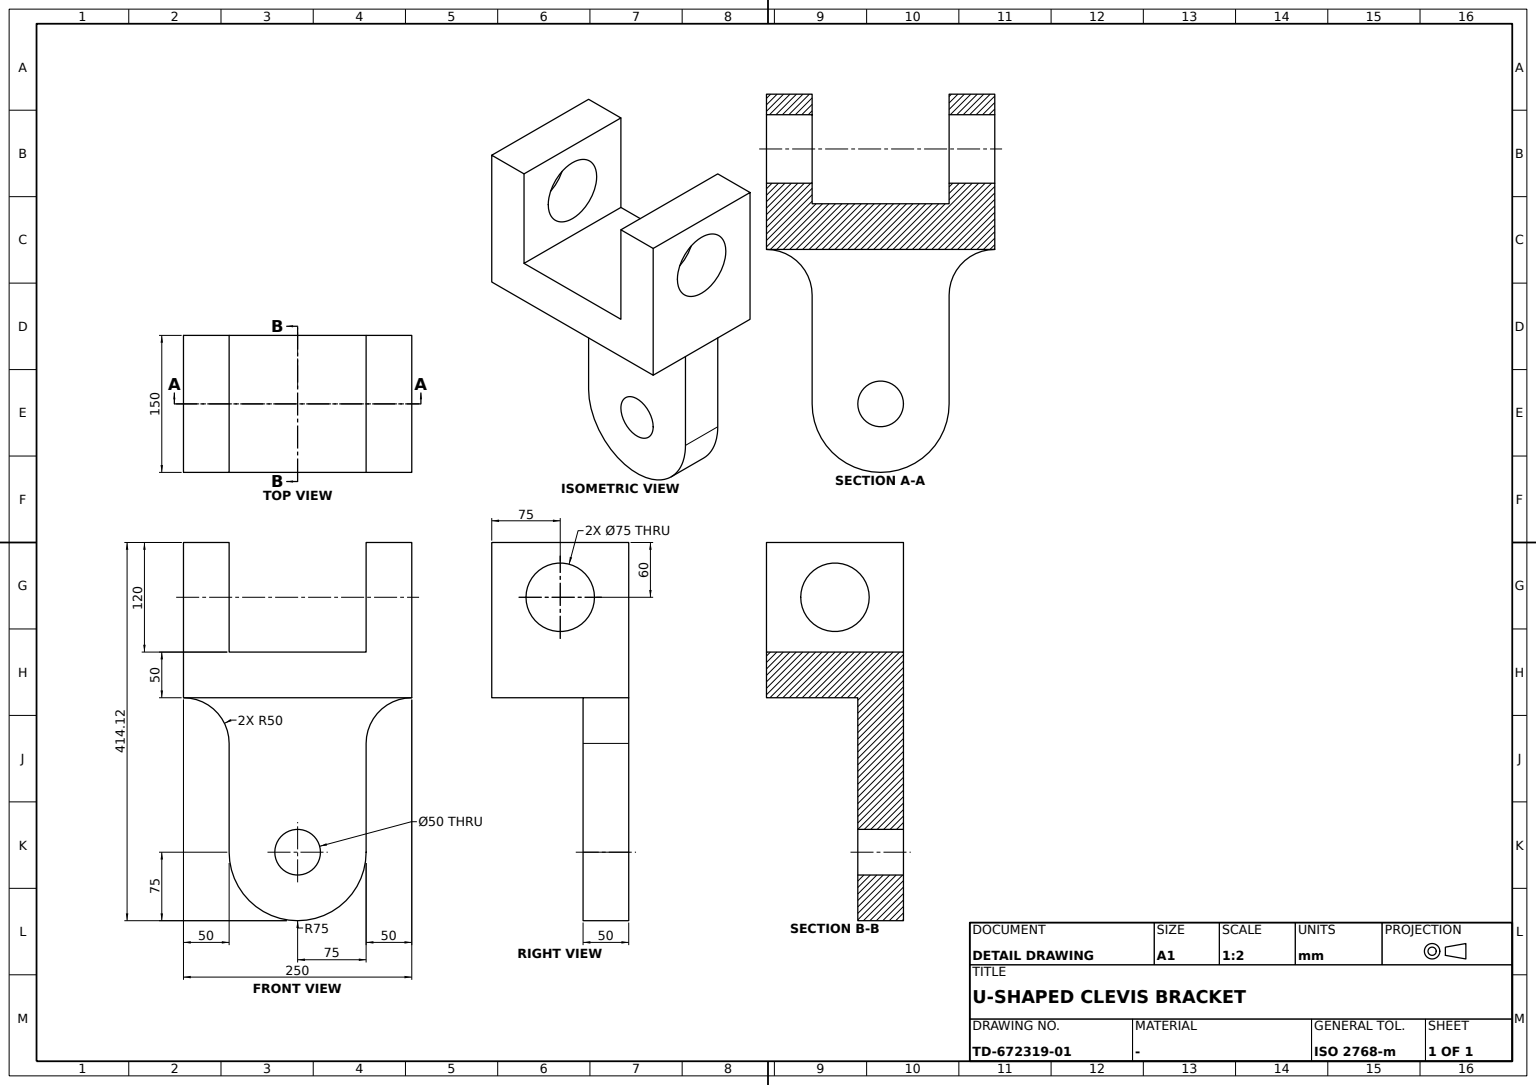
ISO-10303-21;
HEADER;
FILE_DESCRIPTION((''),'2;1');
FILE_NAME('','',(''),(''),'','','');
FILE_SCHEMA(('AUTOMOTIVE_DESIGN'));
ENDSEC;
DATA;
#1=APPLICATION_CONTEXT('');
#2=PRODUCT_CONTEXT('',#1,'mechanical');
#3=PRODUCT('','','',(#2));
#4=PRODUCT_DEFINITION_FORMATION('','',#3);
#5=PRODUCT_DEFINITION_CONTEXT('',#1,'design');
#6=PRODUCT_DEFINITION('','',#4,#5);
#7=PRODUCT_DEFINITION_SHAPE('','',#6);
#8=(LENGTH_UNIT()NAMED_UNIT(*)SI_UNIT(.MILLI.,.METRE.));
#9=(NAMED_UNIT(*)PLANE_ANGLE_UNIT()SI_UNIT($,.RADIAN.));
#10=(NAMED_UNIT(*)SI_UNIT($,.STERADIAN.)SOLID_ANGLE_UNIT());
#11=UNCERTAINTY_MEASURE_WITH_UNIT(LENGTH_MEASURE(1.E-05),#8,'distance_accuracy_value','');
#12=(GEOMETRIC_REPRESENTATION_CONTEXT(3)GLOBAL_UNCERTAINTY_ASSIGNED_CONTEXT((#11))GLOBAL_UNIT_ASSIGNED_CONTEXT((#8,#9,#10))REPRESENTATION_CONTEXT('',''));
#13=CARTESIAN_POINT('',(37.5,75.,60.));
#14=VERTEX_POINT('',#13);
#15=CARTESIAN_POINT('',(-37.5,75.,60.));
#16=VERTEX_POINT('',#15);
#17=CARTESIAN_POINT('',(0.,75.,60.));
#18=DIRECTION('',(0.,1.,0.));
#19=DIRECTION('',(0.,0.,1.));
#20=AXIS2_PLACEMENT_3D('',#17,#18,#19);
#21=CIRCLE('',#20,37.5);
#22=EDGE_CURVE('',#14,#16,#21,.T.);
#23=ORIENTED_EDGE('',*,*,#22,.F.);
#24=CARTESIAN_POINT('',(37.5,125.,60.));
#25=VERTEX_POINT('',#24);
#26=CARTESIAN_POINT('',(37.5,-0.66,60.));
#27=DIRECTION('',(0.,-1.,0.));
#28=VECTOR('',#27,1000.);
#29=LINE('',#26,#28);
#30=EDGE_CURVE('',#25,#14,#29,.T.);
#31=ORIENTED_EDGE('',*,*,#30,.F.);
#32=CARTESIAN_POINT('',(-37.5,125.,60.));
#33=VERTEX_POINT('',#32);
#34=CARTESIAN_POINT('',(0.,125.,60.));
#35=DIRECTION('',(-1.,0.,0.));
#36=AXIS2_PLACEMENT_3D('',#34,#18,#35);
#37=CIRCLE('',#36,37.5);
#38=EDGE_CURVE('',#25,#33,#37,.T.);
#39=ORIENTED_EDGE('',*,*,#38,.T.);
#40=CARTESIAN_POINT('',(-37.5,-0.66,60.));
#41=LINE('',#40,#28);
#42=EDGE_CURVE('',#33,#16,#41,.T.);
#43=ORIENTED_EDGE('',*,*,#42,.T.);
#44=EDGE_LOOP('',(#23,#31,#39,#43));
#45=FACE_OUTER_BOUND('',#44,.T.);
#46=CARTESIAN_POINT('',(0.,-0.66,60.));
#47=AXIS2_PLACEMENT_3D('',#46,#27,#35);
#48=CYLINDRICAL_SURFACE('',#47,37.5);
#49=ADVANCED_FACE('',(#45),#48,.F.);
#50=CARTESIAN_POINT('',(75.,-75.,0.));
#51=VERTEX_POINT('',#50);
#52=CARTESIAN_POINT('',(75.,-75.,120.));
#53=VERTEX_POINT('',#52);
#54=CARTESIAN_POINT('',(75.,-75.,60.));
#55=VECTOR('',#19,1000.);
#56=LINE('',#54,#55);
#57=EDGE_CURVE('',#51,#53,#56,.T.);
#58=ORIENTED_EDGE('',*,*,#57,.F.);
#59=CARTESIAN_POINT('',(-75.,-75.,0.));
#60=VERTEX_POINT('',#59);
#61=CARTESIAN_POINT('',(0.,-75.,0.));
#62=DIRECTION('',(1.,0.,0.));
#63=VECTOR('',#62,1000.);
#64=LINE('',#61,#63);
#65=EDGE_CURVE('',#60,#51,#64,.T.);
#66=ORIENTED_EDGE('',*,*,#65,.F.);
#67=CARTESIAN_POINT('',(-75.,-75.,120.));
#68=VERTEX_POINT('',#67);
#69=CARTESIAN_POINT('',(-75.,-75.,60.));
#70=LINE('',#69,#55);
#71=EDGE_CURVE('',#60,#68,#70,.T.);
#72=ORIENTED_EDGE('',*,*,#71,.T.);
#73=CARTESIAN_POINT('',(0.,-75.,120.));
#74=LINE('',#73,#63);
#75=EDGE_CURVE('',#68,#53,#74,.T.);
#76=ORIENTED_EDGE('',*,*,#75,.T.);
#77=EDGE_LOOP('',(#58,#66,#72,#76));
#78=FACE_OUTER_BOUND('',#77,.T.);
#79=CARTESIAN_POINT('',(-37.5,-75.,60.));
#80=VERTEX_POINT('',#79);
#81=CARTESIAN_POINT('',(37.5,-75.,60.));
#82=VERTEX_POINT('',#81);
#83=CARTESIAN_POINT('',(0.,-75.,60.));
#84=AXIS2_PLACEMENT_3D('',#83,#18,#19);
#85=CIRCLE('',#84,37.5);
#86=EDGE_CURVE('',#80,#82,#85,.T.);
#87=ORIENTED_EDGE('',*,*,#86,.F.);
#88=EDGE_CURVE('',#82,#80,#85,.T.);
#89=ORIENTED_EDGE('',*,*,#88,.F.);
#90=EDGE_LOOP('',(#87,#89));
#91=FACE_BOUND('',#90,.T.);
#92=AXIS2_PLACEMENT_3D('',#61,#18,#19);
#93=PLANE('',#92);
#94=ADVANCED_FACE('',(#78,#91),#93,.T.);
#95=ORIENTED_EDGE('',*,*,#38,.F.);
#96=EDGE_CURVE('',#33,#25,#37,.T.);
#97=ORIENTED_EDGE('',*,*,#96,.F.);
#98=EDGE_LOOP('',(#95,#97));
#99=FACE_BOUND('',#98,.T.);
#100=CARTESIAN_POINT('',(75.,125.,-50.));
#101=VERTEX_POINT('',#100);
#102=CARTESIAN_POINT('',(75.,125.,120.));
#103=VERTEX_POINT('',#102);
#104=CARTESIAN_POINT('',(75.,125.,35.));
#105=LINE('',#104,#55);
#106=EDGE_CURVE('',#101,#103,#105,.T.);
#107=ORIENTED_EDGE('',*,*,#106,.F.);
#108=CARTESIAN_POINT('',(-25.,125.,-50.));
#109=VERTEX_POINT('',#108);
#110=CARTESIAN_POINT('',(25.,125.,-50.));
#111=LINE('',#110,#63);
#112=EDGE_CURVE('',#109,#101,#111,.T.);
#113=ORIENTED_EDGE('',*,*,#112,.F.);
#114=CARTESIAN_POINT('',(-75.,125.,-50.));
#115=VERTEX_POINT('',#114);
#116=CARTESIAN_POINT('',(0.,125.,-50.));
#117=LINE('',#116,#63);
#118=EDGE_CURVE('',#115,#109,#117,.T.);
#119=ORIENTED_EDGE('',*,*,#118,.F.);
#120=CARTESIAN_POINT('',(-75.,125.,120.));
#121=VERTEX_POINT('',#120);
#122=CARTESIAN_POINT('',(-75.,125.,35.));
#123=LINE('',#122,#55);
#124=EDGE_CURVE('',#115,#121,#123,.T.);
#125=ORIENTED_EDGE('',*,*,#124,.T.);
#126=CARTESIAN_POINT('',(0.,125.,120.));
#127=LINE('',#126,#63);
#128=EDGE_CURVE('',#121,#103,#127,.T.);
#129=ORIENTED_EDGE('',*,*,#128,.T.);
#130=EDGE_LOOP('',(#107,#113,#119,#125,#129));
#131=FACE_OUTER_BOUND('',#130,.T.);
#132=DIRECTION('',(0.,0.,-1.));
#133=AXIS2_PLACEMENT_3D('',#126,#27,#132);
#134=PLANE('',#133);
#135=ADVANCED_FACE('',(#99,#131),#134,.F.);
#136=CARTESIAN_POINT('',(75.,75.,0.));
#137=VERTEX_POINT('',#136);
#138=CARTESIAN_POINT('',(75.,0.,0.));
#139=LINE('',#138,#28);
#140=EDGE_CURVE('',#137,#51,#139,.T.);
#141=ORIENTED_EDGE('',*,*,#140,.F.);
#142=CARTESIAN_POINT('',(-75.,75.,0.));
#143=VERTEX_POINT('',#142);
#144=CARTESIAN_POINT('',(0.,75.,0.));
#145=LINE('',#144,#63);
#146=EDGE_CURVE('',#143,#137,#145,.T.);
#147=ORIENTED_EDGE('',*,*,#146,.F.);
#148=CARTESIAN_POINT('',(-75.,0.,0.));
#149=LINE('',#148,#28);
#150=EDGE_CURVE('',#143,#60,#149,.T.);
#151=ORIENTED_EDGE('',*,*,#150,.T.);
#152=ORIENTED_EDGE('',*,*,#65,.T.);
#153=EDGE_LOOP('',(#141,#147,#151,#152));
#154=FACE_OUTER_BOUND('',#153,.T.);
#155=AXIS2_PLACEMENT_3D('',#61,#132,#18);
#156=PLANE('',#155);
#157=ADVANCED_FACE('',(#154),#156,.F.);
#158=CARTESIAN_POINT('',(-25.,-25.,-219.120758));
#159=VERTEX_POINT('',#158);
#160=CARTESIAN_POINT('',(-25.,25.,-219.120758));
#161=VERTEX_POINT('',#160);
#162=CARTESIAN_POINT('',(-25.,0.,-219.120758));
#163=AXIS2_PLACEMENT_3D('',#162,#62,#132);
#164=CIRCLE('',#163,25.);
#165=EDGE_CURVE('',#159,#161,#164,.T.);
#166=ORIENTED_EDGE('',*,*,#165,.T.);
#167=CARTESIAN_POINT('',(-75.,25.,-219.120758));
#168=VERTEX_POINT('',#167);
#169=CARTESIAN_POINT('',(0.,25.,-219.120758));
#170=LINE('',#169,#63);
#171=EDGE_CURVE('',#168,#161,#170,.T.);
#172=ORIENTED_EDGE('',*,*,#171,.F.);
#173=CARTESIAN_POINT('',(-75.,-25.,-219.120758));
#174=VERTEX_POINT('',#173);
#175=CARTESIAN_POINT('',(-75.,0.,-219.120758));
#176=AXIS2_PLACEMENT_3D('',#175,#62,#18);
#177=CIRCLE('',#176,25.);
#178=EDGE_CURVE('',#174,#168,#177,.T.);
#179=ORIENTED_EDGE('',*,*,#178,.F.);
#180=CARTESIAN_POINT('',(0.,-25.,-219.120758));
#181=LINE('',#180,#63);
#182=EDGE_CURVE('',#174,#159,#181,.T.);
#183=ORIENTED_EDGE('',*,*,#182,.T.);
#184=EDGE_LOOP('',(#166,#172,#179,#183));
#185=FACE_OUTER_BOUND('',#184,.T.);
#186=CARTESIAN_POINT('',(0.,0.,-219.120758));
#187=AXIS2_PLACEMENT_3D('',#186,#35,#18);
#188=CYLINDRICAL_SURFACE('',#187,25.);
#189=ADVANCED_FACE('',(#185),#188,.F.);
#190=CARTESIAN_POINT('',(-75.,75.,-219.120758));
#191=VERTEX_POINT('',#190);
#192=CARTESIAN_POINT('',(-25.,75.,-219.120758));
#193=VERTEX_POINT('',#192);
#194=CARTESIAN_POINT('',(0.,75.,-219.120758));
#195=LINE('',#194,#63);
#196=EDGE_CURVE('',#191,#193,#195,.T.);
#197=ORIENTED_EDGE('',*,*,#196,.F.);
#198=CARTESIAN_POINT('',(-75.,75.,-100.));
#199=VERTEX_POINT('',#198);
#200=CARTESIAN_POINT('',(-75.,75.,-159.560379));
#201=LINE('',#200,#55);
#202=EDGE_CURVE('',#191,#199,#201,.T.);
#203=ORIENTED_EDGE('',*,*,#202,.T.);
#204=CARTESIAN_POINT('',(-25.,75.,-100.));
#205=VERTEX_POINT('',#204);
#206=CARTESIAN_POINT('',(-50.,75.,-100.));
#207=LINE('',#206,#63);
#208=EDGE_CURVE('',#199,#205,#207,.T.);
#209=ORIENTED_EDGE('',*,*,#208,.T.);
#210=CARTESIAN_POINT('',(-25.,75.,-159.560379));
#211=LINE('',#210,#55);
#212=EDGE_CURVE('',#193,#205,#211,.T.);
#213=ORIENTED_EDGE('',*,*,#212,.F.);
#214=EDGE_LOOP('',(#197,#203,#209,#213));
#215=FACE_OUTER_BOUND('',#214,.T.);
#216=AXIS2_PLACEMENT_3D('',#194,#18,#19);
#217=PLANE('',#216);
#218=ADVANCED_FACE('',(#215),#217,.T.);
#219=CARTESIAN_POINT('',(-75.,-75.,-219.120758));
#220=VERTEX_POINT('',#219);
#221=CIRCLE('',#176,75.);
#222=EDGE_CURVE('',#220,#191,#221,.T.);
#223=ORIENTED_EDGE('',*,*,#222,.T.);
#224=ORIENTED_EDGE('',*,*,#196,.T.);
#225=CARTESIAN_POINT('',(-25.,-75.,-219.120758));
#226=VERTEX_POINT('',#225);
#227=CIRCLE('',#163,75.);
#228=EDGE_CURVE('',#226,#193,#227,.T.);
#229=ORIENTED_EDGE('',*,*,#228,.F.);
#230=CARTESIAN_POINT('',(-50.,-75.,-219.120758));
#231=LINE('',#230,#63);
#232=EDGE_CURVE('',#220,#226,#231,.T.);
#233=ORIENTED_EDGE('',*,*,#232,.F.);
#234=EDGE_LOOP('',(#223,#224,#229,#233));
#235=FACE_OUTER_BOUND('',#234,.T.);
#236=CYLINDRICAL_SURFACE('',#187,75.);
#237=ADVANCED_FACE('',(#235),#236,.T.);
#238=ORIENTED_EDGE('',*,*,#42,.F.);
#239=ORIENTED_EDGE('',*,*,#96,.T.);
#240=ORIENTED_EDGE('',*,*,#30,.T.);
#241=EDGE_CURVE('',#16,#14,#21,.T.);
#242=ORIENTED_EDGE('',*,*,#241,.F.);
#243=EDGE_LOOP('',(#238,#239,#240,#242));
#244=FACE_OUTER_BOUND('',#243,.T.);
#245=ADVANCED_FACE('',(#244),#48,.F.);
#246=ORIENTED_EDGE('',*,*,#140,.T.);
#247=ORIENTED_EDGE('',*,*,#57,.T.);
#248=CARTESIAN_POINT('',(75.,-125.,120.));
#249=VERTEX_POINT('',#248);
#250=CARTESIAN_POINT('',(75.,-100.,120.));
#251=LINE('',#250,#28);
#252=EDGE_CURVE('',#53,#249,#251,.T.);
#253=ORIENTED_EDGE('',*,*,#252,.T.);
#254=CARTESIAN_POINT('',(75.,-125.,-50.));
#255=VERTEX_POINT('',#254);
#256=CARTESIAN_POINT('',(75.,-125.,35.));
#257=VECTOR('',#132,1000.);
#258=LINE('',#256,#257);
#259=EDGE_CURVE('',#249,#255,#258,.T.);
#260=ORIENTED_EDGE('',*,*,#259,.T.);
#261=CARTESIAN_POINT('',(75.,0.,-50.));
#262=VECTOR('',#18,1000.);
#263=LINE('',#261,#262);
#264=EDGE_CURVE('',#255,#101,#263,.T.);
#265=ORIENTED_EDGE('',*,*,#264,.T.);
#266=ORIENTED_EDGE('',*,*,#106,.T.);
#267=CARTESIAN_POINT('',(75.,75.,120.));
#268=VERTEX_POINT('',#267);
#269=CARTESIAN_POINT('',(75.,100.,120.));
#270=LINE('',#269,#28);
#271=EDGE_CURVE('',#103,#268,#270,.T.);
#272=ORIENTED_EDGE('',*,*,#271,.T.);
#273=CARTESIAN_POINT('',(75.,75.,60.));
#274=LINE('',#273,#257);
#275=EDGE_CURVE('',#268,#137,#274,.T.);
#276=ORIENTED_EDGE('',*,*,#275,.T.);
#277=EDGE_LOOP('',(#246,#247,#253,#260,#265,#266,#272,#276));
#278=FACE_OUTER_BOUND('',#277,.T.);
#279=AXIS2_PLACEMENT_3D('',#138,#62,#18);
#280=PLANE('',#279);
#281=ADVANCED_FACE('',(#278),#280,.T.);
#282=ORIENTED_EDGE('',*,*,#271,.F.);
#283=ORIENTED_EDGE('',*,*,#128,.F.);
#284=CARTESIAN_POINT('',(-75.,75.,120.));
#285=VERTEX_POINT('',#284);
#286=CARTESIAN_POINT('',(-75.,100.,120.));
#287=LINE('',#286,#28);
#288=EDGE_CURVE('',#121,#285,#287,.T.);
#289=ORIENTED_EDGE('',*,*,#288,.T.);
#290=CARTESIAN_POINT('',(0.,75.,120.));
#291=LINE('',#290,#63);
#292=EDGE_CURVE('',#285,#268,#291,.T.);
#293=ORIENTED_EDGE('',*,*,#292,.T.);
#294=EDGE_LOOP('',(#282,#283,#289,#293));
#295=FACE_OUTER_BOUND('',#294,.T.);
#296=AXIS2_PLACEMENT_3D('',#73,#19,#27);
#297=PLANE('',#296);
#298=ADVANCED_FACE('',(#295),#297,.T.);
#299=CARTESIAN_POINT('',(-75.,-125.,120.));
#300=VERTEX_POINT('',#299);
#301=CARTESIAN_POINT('',(-75.,-100.,120.));
#302=LINE('',#301,#28);
#303=EDGE_CURVE('',#68,#300,#302,.T.);
#304=ORIENTED_EDGE('',*,*,#303,.F.);
#305=ORIENTED_EDGE('',*,*,#71,.F.);
#306=ORIENTED_EDGE('',*,*,#150,.F.);
#307=CARTESIAN_POINT('',(-75.,75.,60.));
#308=LINE('',#307,#257);
#309=EDGE_CURVE('',#285,#143,#308,.T.);
#310=ORIENTED_EDGE('',*,*,#309,.F.);
#311=ORIENTED_EDGE('',*,*,#288,.F.);
#312=ORIENTED_EDGE('',*,*,#124,.F.);
#313=CARTESIAN_POINT('',(-75.,125.,-100.));
#314=AXIS2_PLACEMENT_3D('',#313,#35,#18);
#315=CIRCLE('',#314,50.);
#316=EDGE_CURVE('',#199,#115,#315,.T.);
#317=ORIENTED_EDGE('',*,*,#316,.F.);
#318=ORIENTED_EDGE('',*,*,#202,.F.);
#319=ORIENTED_EDGE('',*,*,#222,.F.);
#320=CARTESIAN_POINT('',(-75.,-75.,-100.));
#321=VERTEX_POINT('',#320);
#322=CARTESIAN_POINT('',(-75.,-75.,-159.560379));
#323=LINE('',#322,#257);
#324=EDGE_CURVE('',#321,#220,#323,.T.);
#325=ORIENTED_EDGE('',*,*,#324,.F.);
#326=CARTESIAN_POINT('',(-75.,-125.,-50.));
#327=VERTEX_POINT('',#326);
#328=CARTESIAN_POINT('',(-75.,-125.,-100.));
#329=AXIS2_PLACEMENT_3D('',#328,#35,#18);
#330=CIRCLE('',#329,50.);
#331=EDGE_CURVE('',#327,#321,#330,.T.);
#332=ORIENTED_EDGE('',*,*,#331,.F.);
#333=CARTESIAN_POINT('',(-75.,-125.,35.));
#334=LINE('',#333,#257);
#335=EDGE_CURVE('',#300,#327,#334,.T.);
#336=ORIENTED_EDGE('',*,*,#335,.F.);
#337=EDGE_LOOP('',(#304,#305,#306,#310,#311,#312,#317,#318,#319,#325,#332,#336));
#338=FACE_OUTER_BOUND('',#337,.T.);
#339=ORIENTED_EDGE('',*,*,#178,.T.);
#340=EDGE_CURVE('',#168,#174,#177,.T.);
#341=ORIENTED_EDGE('',*,*,#340,.T.);
#342=EDGE_LOOP('',(#339,#341));
#343=FACE_BOUND('',#342,.T.);
#344=AXIS2_PLACEMENT_3D('',#148,#62,#18);
#345=PLANE('',#344);
#346=ADVANCED_FACE('',(#338,#343),#345,.F.);
#347=ORIENTED_EDGE('',*,*,#22,.T.);
#348=ORIENTED_EDGE('',*,*,#241,.T.);
#349=EDGE_LOOP('',(#347,#348));
#350=FACE_BOUND('',#349,.T.);
#351=ORIENTED_EDGE('',*,*,#309,.T.);
#352=ORIENTED_EDGE('',*,*,#146,.T.);
#353=ORIENTED_EDGE('',*,*,#275,.F.);
#354=ORIENTED_EDGE('',*,*,#292,.F.);
#355=EDGE_LOOP('',(#351,#352,#353,#354));
#356=FACE_OUTER_BOUND('',#355,.T.);
#357=ADVANCED_FACE('',(#350,#356),#217,.F.);
#358=CARTESIAN_POINT('',(-25.,-75.,-100.));
#359=VERTEX_POINT('',#358);
#360=CARTESIAN_POINT('',(0.,-75.,-100.));
#361=LINE('',#360,#63);
#362=EDGE_CURVE('',#321,#359,#361,.T.);
#363=ORIENTED_EDGE('',*,*,#362,.F.);
#364=ORIENTED_EDGE('',*,*,#324,.T.);
#365=ORIENTED_EDGE('',*,*,#232,.T.);
#366=CARTESIAN_POINT('',(-25.,-75.,-159.560379));
#367=LINE('',#366,#55);
#368=EDGE_CURVE('',#226,#359,#367,.T.);
#369=ORIENTED_EDGE('',*,*,#368,.T.);
#370=EDGE_LOOP('',(#363,#364,#365,#369));
#371=FACE_OUTER_BOUND('',#370,.T.);
#372=ADVANCED_FACE('',(#371),#93,.F.);
#373=ORIENTED_EDGE('',*,*,#264,.F.);
#374=CARTESIAN_POINT('',(-25.,-125.,-50.));
#375=VERTEX_POINT('',#374);
#376=CARTESIAN_POINT('',(25.,-125.,-50.));
#377=LINE('',#376,#63);
#378=EDGE_CURVE('',#375,#255,#377,.T.);
#379=ORIENTED_EDGE('',*,*,#378,.F.);
#380=CARTESIAN_POINT('',(-25.,0.,-50.));
#381=LINE('',#380,#262);
#382=EDGE_CURVE('',#375,#109,#381,.T.);
#383=ORIENTED_EDGE('',*,*,#382,.T.);
#384=ORIENTED_EDGE('',*,*,#112,.T.);
#385=EDGE_LOOP('',(#373,#379,#383,#384));
#386=FACE_OUTER_BOUND('',#385,.T.);
#387=CARTESIAN_POINT('',(102.805157,-75.,-50.));
#388=AXIS2_PLACEMENT_3D('',#387,#132,#35);
#389=PLANE('',#388);
#390=ADVANCED_FACE('',(#386),#389,.T.);
#391=CARTESIAN_POINT('',(37.5,-125.,60.));
#392=VERTEX_POINT('',#391);
#393=CARTESIAN_POINT('',(-37.5,-125.,60.));
#394=VERTEX_POINT('',#393);
#395=CARTESIAN_POINT('',(0.,-125.,60.));
#396=AXIS2_PLACEMENT_3D('',#395,#27,#132);
#397=CIRCLE('',#396,37.5);
#398=EDGE_CURVE('',#392,#394,#397,.T.);
#399=ORIENTED_EDGE('',*,*,#398,.T.);
#400=EDGE_CURVE('',#80,#394,#41,.T.);
#401=ORIENTED_EDGE('',*,*,#400,.F.);
#402=ORIENTED_EDGE('',*,*,#86,.T.);
#403=EDGE_CURVE('',#82,#392,#29,.T.);
#404=ORIENTED_EDGE('',*,*,#403,.T.);
#405=EDGE_LOOP('',(#399,#401,#402,#404));
#406=FACE_OUTER_BOUND('',#405,.T.);
#407=ADVANCED_FACE('',(#406),#48,.F.);
#408=ORIENTED_EDGE('',*,*,#208,.F.);
#409=ORIENTED_EDGE('',*,*,#316,.T.);
#410=ORIENTED_EDGE('',*,*,#118,.T.);
#411=CARTESIAN_POINT('',(-25.,125.,-100.));
#412=AXIS2_PLACEMENT_3D('',#411,#62,#132);
#413=CIRCLE('',#412,50.);
#414=EDGE_CURVE('',#109,#205,#413,.T.);
#415=ORIENTED_EDGE('',*,*,#414,.T.);
#416=EDGE_LOOP('',(#408,#409,#410,#415));
#417=FACE_OUTER_BOUND('',#416,.T.);
#418=CARTESIAN_POINT('',(0.,125.,-100.));
#419=AXIS2_PLACEMENT_3D('',#418,#35,#18);
#420=CYLINDRICAL_SURFACE('',#419,50.);
#421=ADVANCED_FACE('',(#417),#420,.F.);
#422=ORIENTED_EDGE('',*,*,#88,.T.);
#423=ORIENTED_EDGE('',*,*,#400,.T.);
#424=EDGE_CURVE('',#394,#392,#397,.T.);
#425=ORIENTED_EDGE('',*,*,#424,.T.);
#426=ORIENTED_EDGE('',*,*,#403,.F.);
#427=EDGE_LOOP('',(#422,#423,#425,#426));
#428=FACE_OUTER_BOUND('',#427,.T.);
#429=ADVANCED_FACE('',(#428),#48,.F.);
#430=ORIENTED_EDGE('',*,*,#362,.T.);
#431=CARTESIAN_POINT('',(-25.,-125.,-100.));
#432=AXIS2_PLACEMENT_3D('',#431,#62,#132);
#433=CIRCLE('',#432,50.);
#434=EDGE_CURVE('',#359,#375,#433,.T.);
#435=ORIENTED_EDGE('',*,*,#434,.T.);
#436=CARTESIAN_POINT('',(-50.,-125.,-50.));
#437=LINE('',#436,#63);
#438=EDGE_CURVE('',#327,#375,#437,.T.);
#439=ORIENTED_EDGE('',*,*,#438,.F.);
#440=ORIENTED_EDGE('',*,*,#331,.T.);
#441=EDGE_LOOP('',(#430,#435,#439,#440));
#442=FACE_OUTER_BOUND('',#441,.T.);
#443=CARTESIAN_POINT('',(0.,-125.,-100.));
#444=AXIS2_PLACEMENT_3D('',#443,#35,#18);
#445=CYLINDRICAL_SURFACE('',#444,50.);
#446=ADVANCED_FACE('',(#442),#445,.F.);
#447=ORIENTED_EDGE('',*,*,#252,.F.);
#448=ORIENTED_EDGE('',*,*,#75,.F.);
#449=ORIENTED_EDGE('',*,*,#303,.T.);
#450=CARTESIAN_POINT('',(0.,-125.,120.));
#451=LINE('',#450,#63);
#452=EDGE_CURVE('',#300,#249,#451,.T.);
#453=ORIENTED_EDGE('',*,*,#452,.T.);
#454=EDGE_LOOP('',(#447,#448,#449,#453));
#455=FACE_OUTER_BOUND('',#454,.T.);
#456=ADVANCED_FACE('',(#455),#297,.T.);
#457=EDGE_CURVE('',#161,#159,#164,.T.);
#458=ORIENTED_EDGE('',*,*,#457,.T.);
#459=ORIENTED_EDGE('',*,*,#182,.F.);
#460=ORIENTED_EDGE('',*,*,#340,.F.);
#461=ORIENTED_EDGE('',*,*,#171,.T.);
#462=EDGE_LOOP('',(#458,#459,#460,#461));
#463=FACE_OUTER_BOUND('',#462,.T.);
#464=ADVANCED_FACE('',(#463),#188,.F.);
#465=ORIENTED_EDGE('',*,*,#414,.F.);
#466=ORIENTED_EDGE('',*,*,#382,.F.);
#467=ORIENTED_EDGE('',*,*,#434,.F.);
#468=ORIENTED_EDGE('',*,*,#368,.F.);
#469=ORIENTED_EDGE('',*,*,#228,.T.);
#470=ORIENTED_EDGE('',*,*,#212,.T.);
#471=EDGE_LOOP('',(#465,#466,#467,#468,#469,#470));
#472=FACE_OUTER_BOUND('',#471,.T.);
#473=ORIENTED_EDGE('',*,*,#457,.F.);
#474=ORIENTED_EDGE('',*,*,#165,.F.);
#475=EDGE_LOOP('',(#473,#474));
#476=FACE_BOUND('',#475,.T.);
#477=CARTESIAN_POINT('',(-25.,-75.,-50.));
#478=AXIS2_PLACEMENT_3D('',#477,#62,#132);
#479=PLANE('',#478);
#480=ADVANCED_FACE('',(#472,#476),#479,.T.);
#481=ORIENTED_EDGE('',*,*,#424,.F.);
#482=ORIENTED_EDGE('',*,*,#398,.F.);
#483=EDGE_LOOP('',(#481,#482));
#484=FACE_BOUND('',#483,.T.);
#485=ORIENTED_EDGE('',*,*,#259,.F.);
#486=ORIENTED_EDGE('',*,*,#452,.F.);
#487=ORIENTED_EDGE('',*,*,#335,.T.);
#488=ORIENTED_EDGE('',*,*,#438,.T.);
#489=ORIENTED_EDGE('',*,*,#378,.T.);
#490=EDGE_LOOP('',(#485,#486,#487,#488,#489));
#491=FACE_OUTER_BOUND('',#490,.T.);
#492=AXIS2_PLACEMENT_3D('',#450,#27,#132);
#493=PLANE('',#492);
#494=ADVANCED_FACE('',(#484,#491),#493,.T.);
#495=CLOSED_SHELL('',(#49,#94,#135,#157,#189,#218,#237,#245,#281,#298,#346,#357,#372,#390,#407,#421,#429,#446,#456,#464,#480,#494));
#496=MANIFOLD_SOLID_BREP('',#495);
#497=ADVANCED_BREP_SHAPE_REPRESENTATION('',(#496),#12);
#498=SHAPE_DEFINITION_REPRESENTATION(#7,#497);
ENDSEC;
END-ISO-10303-21;
